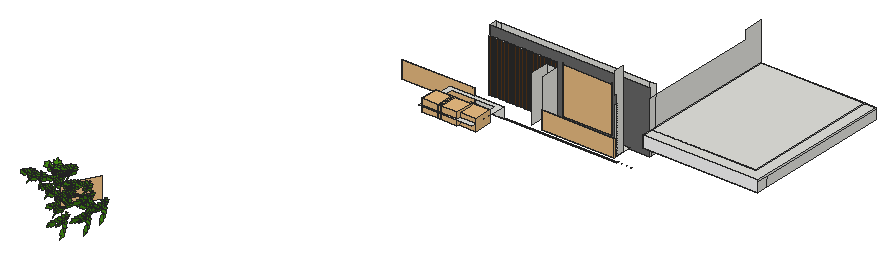
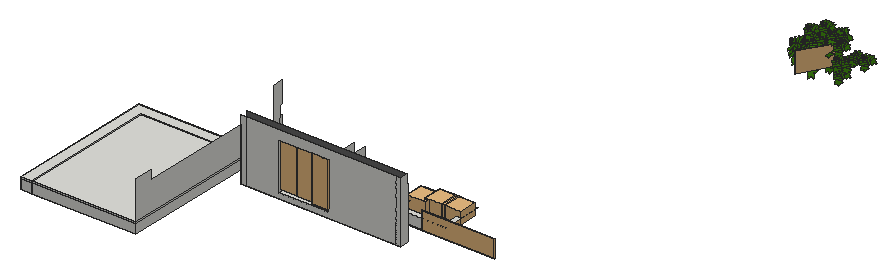
# SketchUp Ruby script. Lengths in inches.
U = 1.inch
M = Sketchup.active_model
def pt(a) = Geom::Point3d.new(a.map { |v| v * U })
def face(e, loops, mat)
  f = e.add_face(loops[0].map { |a| pt(a) })
  loops[1..].each { |l| e.add_face(l.map { |a| pt(a) }).erase! }
  f.material = f.back_material = mat if mat
  f
end
# faces: each face lists its corners as indices into pts; further lists are holes
def faces(e, pts, list, mat = nil) = list.each { |f| face(e, (f[0].is_a?(Array) ? f : [f]).map { |l| l.map { |i| pts[i] } }, mat) }
# xy, xz, yz: faces in a plane at the given z, y or x. An outline is a flat list of corners, or four numbers for a rectangle; further outlines are holes
def ring(l) = l.size == 4 ? [[l[0], l[1]], [l[2], l[1]], [l[2], l[3]], [l[0], l[3]]] : l.each_slice(2).to_a
def flat(e, list, mat, &to3) = list.each { |f| face(e, (f[0].is_a?(Array) ? f : [f]).map { |l| ring(l).map { |u, v| to3.(u, v) } }, mat) }
def xy(e, z, list, mat = nil) = flat(e, list, mat) { |x, y| [x, y, z] }
def xz(e, y, list, mat = nil) = flat(e, list, mat) { |x, z| [x, y, z] }
def yz(e, x, list, mat = nil) = flat(e, list, mat) { |y, z| [x, y, z] }
def lines(e, pts, list) = list.each { |a, b| e.add_line(pt(pts[a]), pt(pts[b])) }
# prism: a flat outline (further loops are holes) pulled along v
def prism(e, loops, v, mat = nil)
  f = face(e, loops, mat); d = Geom::Vector3d.new(v.map { |x| x * U })
  f.pushpull(f.normal.samedirection?(d) ? d.length : -d.length)
end
def box(e, o, s, mat = nil) = prism(e, [[o, [o[0] + s[0], o[1], o[2]], [o[0] + s[0], o[1] + s[1], o[2]], [o[0], o[1] + s[1], o[2]]]], [0, 0, s[2]], mat)
def at(x, y, z, deg = 0) = Geom::Transformation.translation(pt([x, y, z])) * Geom::Transformation.rotation(ORIGIN, Z_AXIS, deg.degrees)
def axes(o, x, y, z) = Geom::Transformation.new([*x, 0, *y, 0, *z, 0, *pt(o).to_a, 1])
def part(name) = M.definitions.add(name)
# library, detail: a bought-in or finely detailed component or shape, given as its bounding box
def library(name, o, s) = part(name).tap { |d| box(d.entities, o, s) }
def detail(e, o, s) = box(e.add_group.entities, o, s)
def put(e, d, t, mat = nil) = e.add_instance(d, t).tap { |i| i.material = mat if mat }
def group(e, t, mat = nil) = e.add_group.tap { |g| g.transformation = t; g.material = mat if mat }.entities
root = M.entities
M.materials.add("Material~3").color = [123, 113, 102]
M.materials.add("[0030_OldLace]").color = [86, 53, 24]
M.materials.add("[0128_White]").color = [255, 255, 255]
M.materials.add("[Slate Light Tile]").color = [104, 104, 104]
M.materials.add("[Wood Veneer 01]").color = [120, 70, 37]
M.materials.add("hojas").color = [70, 150, 19]
c1 = part("rama-acacia")
p = [[-13.53,0.69,-1.07],[-13.38,0.86,-0.98],[-13.61,0.85,-1.06],[-14.07,0.85,-1.21],[-15.17,0.86,-1.58],[-15.95,0.92,-1.83],
  [-16.01,1,-1.83],[-16.01,1.17,-1.78],[-16.07,1.93,-1.6],[-16.4,2.73,-1.5],[-16.65,3.06,-1.5],[-17.13,4.01,-1.41],
  [-17.78,4.7,-1.44],[-18.28,5.07,-1.51],[-18.57,5.18,-1.58],[-18.91,5.47,-1.62],[-19.07,5.48,-1.67],[-19.35,5.61,-1.73],
  [-19.51,5.64,-1.78],[-19.38,5.57,-1.75],[-19.33,5.5,-1.75],[-19.31,5.23,-1.82],[-19.38,5.08,-1.89],[-19.41,4.84,-1.96],
  [-19.36,4.59,-2.01],[-19.43,4.55,-2.04],[-19.36,4.15,-2.125],[-19.21,3.7,-2.19],[-18.875,3.1,-2.24],[-18.61,2.78,-2.24],
  [-17.83,2.19,-2.13],[-17.4375,1.85,-2.09],[-17.04,1.49,-2.05],[-16.61,1.24,-1.97],[-16.17,1.0625,-1.87],[-16.06,0.95,-1.86],
  [-16.06,0.91,-1.87],[-16.32,0.9,-1.96],[-16.7,0.88,-2.1],[-17.05,0.91,-2.21],[-17.61,1.15,-2.33],[-18.06,1.29,-2.45],
  [-18.88,1.53,-2.67],[-20.25,1.46,-3.15],[-20.59,1.49,-3.26],[-20.79,1.37,-3.36],[-21.08,1.2,-3.5],[-21.28,1.22,-3.5625],
  [-21.48,0.94,-3.71],[-21.79,0.5,-3.93],[-22.02,0.17,-4.1],[-22.11,0.05,-4.16],[-22.21,-0.02,-4.21],[-22.375,-0.05,-4.28],
  [-22.375,-0.07,-4.28],[-22.18,-0.09,-4.22],[-22.11,-0.07,-4.19],[-21.78,-0.1,-4.09],[-21.6,-0.18,-4.05],[-21.52,-0.27,-4.04],
  [-21.33,-0.33,-4],[-20.94,-0.54,-3.92],[-20.6875,-0.63,-3.86],[-20.54,-0.68,-3.82],[-20.42,-0.67,-3.78],[-20.09,-0.46,-3.61],
  [-19.8,-0.24,-3.45],[-19.21,-0.02,-3.19],[-18.48,0.08,-2.92],[-17.72,0.38,-2.58],[-17.4,0.5,-2.4375],[-16.93,0.75,-2.21],
  [-16.78,0.8,-2.15],[-16.1,0.83,-1.91],[-16.0625,0.81,-1.9],[-16.08,0.77,-1.91],[-16.27,0.72,-1.99],[-16.88,0.39,-2.29],
  [-17.1875,0.15,-2.46],[-17.27,0.02,-2.52],[-17.94,-0.52,-2.89],[-17.94,-0.59,-2.91],[-18.08,-0.68,-2.99],[-18.13,-0.86,-3.05],
  [-18.56,-1.55,-3.38],[-18.71,-2.11,-3.58],[-18.79,-2.61,-3.74],[-18.86,-2.84,-3.83],[-18.87,-3.07,-3.89],[-18.84,-3.22,-3.92],
  [-18.8,-3.26,-3.92],[-18.76,-3.47,-3.96],[-18.76,-3.6,-4],[-18.67,-3.8,-4.02],[-18.61,-3.92,-4.04],[-18.58,-4.11,-4.07],
  [-18.53,-4.18,-4.08],[-18.58,-4.35,-4.14],[-18.65,-4.43,-4.18],[-18.72,-4.51,-4.23],[-18.8125,-4.51,-4.26],[-18.8125,-4.53,-4.26],
  [-18.72,-4.54,-4.24],[-18.66,-4.49,-4.21],[-18.58,-4.43,-4.16],[-18.35,-4.23,-4.03],[-18.32,-4.17,-4],[-18.22,-4.125,-3.95],
  [-18.1,-4,-3.88],[-17.79,-3.72,-3.7],[-17.68,-3.51,-3.61],[-17.32,-3.13,-3.38],[-17.24,-2.94,-3.31],[-16.78,-2.12,-2.93],
  [-16.48,-1.78,-2.73],[-16.3,-1.28,-2.54],[-16.05,-0.75,-2.3125],[-15.89,-0.2,-2.11],[-15.89,0.39,-1.95],[-15.96,0.79,-1.87],
  [-15.91,0.82,-1.84],[-15.27,0.8,-1.63],[-14.18,0.76,-1.27],[-13.78,0.73,-1.15],[-13.78,0.67,-1.16],[-14.23,0.54,-1.35],
  [-14.65,0.33,-1.55],[-14.97,0.02,-1.74],[-15.25,-0.36,-1.9375],[-15.57,-0.72,-2.14],[-15.96,-1.64,-2.52],[-16.2,-2.51,-2.84],
  [-16.2,-3.12,-3],[-16.14,-3.41,-3.06],[-16.1,-3.75,-3.14],[-16.1,-4.09,-3.23],[-16.2,-4.25,-3.3],[-16.2,-4.28,-3.3125],
  [-16.08,-4.19,-3.24],[-15.98,-4.08,-3.18],[-15.96,-3.94,-3.14],[-15.96,-3.8125,-3.1],[-15.9,-3.72,-3.06],[-15.68,-3.55,-2.9375],
  [-15.51,-3.49,-2.86],[-15.3,-3.33,-2.75],[-15.23,-3.17,-2.68],[-15.01,-3.03,-2.57],[-14.875,-2.83,-2.47],[-14.6,-2.59,-2.3125],
  [-14.4,-2.27,-2.16],[-14.12,-1.6,-1.89],[-13.91,-1.1,-1.68],[-13.67,-0.83,-1.53],[-13.53,-0.45,-1.38],[-13.53,0.67,-1.08],
  [-12.41,6.01,0.65],[-12.44,6.14,0.68],[-12.41,6.29,0.73],[-12.43,6.29,0.73],[-12.44,6.26,0.72],[-12.47,6.15,0.68],
  [-12.49,6.07,0.66],[-12.57,5.75,0.55],[-12.67,5.36,0.43],[-12.79,4.875,0.28],[-12.83,4.52,0.18],[-12.83,3.99,0.04],
  [-12.73,3.11,-0.18],[-12.58,2.52,-0.3125],[-12.3,1.97,-0.41],[-11.88,1.51,-0.46],[-11.37,1.0625,-0.48],[-10.75,0.75,-0.45],
  [-10.75,0.68,-0.47],[-12.55,0.7,-0.79],[-13.21,0.79,-0.89],[-13.2,0.67,-0.92],[-12.56,0.62,-0.82],[-11.15,0.56,-0.58],
  [-10.79,0.54,-0.52],[-10.72,0.52,-0.51],[-10.72,0.5,-0.52],[-10.87,0.47,-0.55],[-11.14,0.41,-0.62],[-11.39,0.27,-0.7],
  [-11.625,-0.01,-0.82],[-11.8,-0.43,-0.96],[-11.83,-0.57,-1],[-12.02,-1.08,-1.17],[-12.1,-1.39,-1.27],[-12.17,-1.95,-1.4375],
  [-12.17,-2.77,-1.65],[-12.09,-3.59,-1.86],[-11.86,-4.26,-2],[-11.8125,-4.4,-2.03],[-11.84,-4.49,-2.05],[-11.91,-4.6,-2.1],
  [-11.97,-4.65,-2.12],[-11.98,-4.67,-2.13],[-11.92,-4.65,-2.11],[-11.84,-4.59,-2.08],[-11.77,-4.52,-2.05],[-11.74,-4.47,-2.03],
  [-11.37,-4.3125,-1.92],[-10.95,-4.0625,-1.78],[-10.82,-3.89,-1.71],[-10.64,-3.57,-1.59],[-10.41,-3.05,-1.41],[-10.27,-2.73,-1.3],
  [-10.07,-1.88,-1.03],[-10.15,-0.71,-0.73],[-10.31,-0.1,-0.6],[-10.5,0.4,-0.5],[-10.5,0.48,-0.48],[-10.44,0.53,-0.45],
  [-10.39,0.64,-0.42],[-10.52,0.73,-0.42],[-10.44,0.93,-0.35],[-10.44,1.2,-0.28],[-10.32,1.47,-0.18],[-10.48,2.6875,0.12],
  [-10.43,2.96,0.2],[-10.75,3.87,0.38],[-11.26,4.93,0.57],[-11.8,5.54,0.64],[-12.37,5.93,0.64],[-7.78,0.19,-0.06],
  [-7.78,0.25,-0.04],[-7.75,0.39,0],[-7.89,0.4,-0.02],[-7.96,0.46,-0.02],[-7.96,0.49,-0.01],[-7.76,0.62,0.06],
  [-7.53,0.99,0.2],[-7.31,1.78,0.45],[-7.31,2.74,0.71],[-7.63,3.6875,0.9],[-8.02,4.57,1.07],[-8.66,5.23,1.13],
  [-8.83,5.4,1.14],[-8.92,5.54,1.16],[-9.1,5.64,1.16],[-9.08,5.6,1.15],[-9.02,5.56,1.15],[-8.94,5.46,1.14],
  [-8.9,5.37,1.12],[-8.9375,5.25,1.08],[-9.14,4.92,0.96],[-9.31,4.5625,0.83],[-9.39,3.73,0.6],[-9.44,2.76,0.32],
  [-9.23,1.59,0.05],[-8.82,0.9,-0.06],[-8.36,0.59,-0.0625],[-8.14,0.51,-0.04],[-8.05,0.48,-0.03],[-8.05,0.46,-0.04],
  [-8.12,0.43,-0.06],[-10.1,0.49,-0.4],[-8.22,0.3125,-0.11],[-8.22,0.25,-0.125],[-8.53,0.13,-0.21],[-8.8,-0.16,-0.34],
  [-8.96,-0.61,-0.49],[-8.96,-0.87,-0.56],[-9.16,-1.42,-0.74],[-9.13,-1.77,-0.83],[-9.09,-1.83,-0.84],[-9.125,-1.92,-0.87],
  [-9.125,-2.13,-0.93],[-9.08,-2.23,-0.95],[-9.15,-2.39,-1],[-9.11,-2.67,-1.07],[-9.03,-2.86,-1.11],[-9.07,-3.03,-1.16],
  [-8.97,-3.23,-1.19],[-8.93,-3.44,-1.24],[-8.93,-3.71,-1.32],[-8.79,-4.05,-1.38],[-8.7,-4.25,-1.42],[-8.7,-4.39,-1.46],
  [-8.76,-4.53,-1.5],[-8.77,-4.65,-1.54],[-8.64,-4.55,-1.49],[-8.27,-4.22,-1.33],[-8.1875,-4.06,-1.27],[-8.07,-3.98,-1.23],
  [-7.98,-3.79,-1.17],[-7.79,-3.59,-1.08],[-7.64,-3.3,-0.97],[-7.64,-3.25,-0.96],[-7.59,-3.21,-0.9375],[-7.52,-2.93,-0.85],
  [-7.52,-2.85,-0.83],[-7.47,-2.81,-0.81],[-7.3,-2.09,-0.59],[-7.32,-2.01,-0.57],[-7.27,-1.95,-0.54],[-7.1875,-1.57,-0.42],
  [-7.17,-1.46,-0.39],[-7.17,-1.16,-0.3125],[-7.23,-0.61,-0.17],[-7.49,-0.15,-0.1],[-13.39,-0.07,-1.23],[-13.39,0.25,-1.14],
  [-13.49,0.5625,-1.09],[-13.8,1.01,-1.08],[-13.61,0.91,-1.04],[-13.38,0.92,-0.96],[-13.32,1.03,-0.91],[-13.32,1.35,-0.82],
  [-13.28,1.49,-0.77],[-13.28,1.99,-0.64],[-13.44,2.67,-0.51],[-13.72,3.31,-0.43],[-13.93,3.71,-0.4],[-14.1,4.39,-0.27],
  [-14.5625,5.06,-0.25],[-14.89,5.62,-0.21],[-15.33,6.1,-0.23],[-15.65,6.8,-0.15],[-15.79,6.89,-0.18],[-15.61,6.52,-0.22],
  [-15.51,6.32,-0.24],[-15.45,6.28,-0.23],[-15.52,6,-0.32],[-15.63,5.6875,-0.45],[-15.77,4.97,-0.68],[-15.7,4.25,-0.85],
  [-15.46,3,-1.11],[-15,2.03,-1.21],[-14.3,1.29,-1.17],[-4.5625,0.33,0.09],[-4.22,0.49,0.13],[-4,0.7,0.1875],
  [-3.86,0.99,0.26],[-3.77,1.41,0.38],[-3.7,1.73,0.46],[-3.77,1.99,0.53],[-3.85,2.17,0.58],[-3.88,2.57,0.6875],
  [-3.98,2.9,0.78],[-4.0625,2.97,0.8],[-4.1,3.14,0.84],[-4.1875,3.25,0.87],[-4.27,3.55,0.95],[-4.31,3.71,0.99],
  [-4.42,3.9,1.04],[-4.625,4.2,1.125],[-4.72,4.39,1.18],[-4.89,4.57,1.23],[-4.98,4.73,1.27],[-5,4.72,1.26],
  [-5.01,4.51,1.21],[-4.96,4.32,1.16],[-4.97,4.27,1.14],[-5.14,3.78,1.01],[-5.3,3.39,0.91],[-5.44,2.76,0.74],
  [-5.5,2.09,0.56],[-5.57,1.78,0.48],[-5.57,1.42,0.38],[-5.57,1.09,0.29],[-5.47,0.72,0.19],[-5.22,0.44,0.12],
  [-4.93,0.27,0.07],[-4.76,0.22,0.06],[-4.76,0.18,0.05],[-4.83,0.16,0.04],[-5.26,0,0],[-5.34,-0.04,-0.01],
  [-5.47,-0.22,-0.06],[-5.51,-0.6,-0.16],[-5.42,-1.09,-0.29],[-5.28,-1.49,-0.4],[-5.21,-1.87,-0.5],[-5.11,-2.15,-0.57],
  [-5.08,-2.34,-0.63],[-5.01,-2.47,-0.66],[-4.96,-2.69,-0.72],[-4.86,-2.9375,-0.79],[-4.84,-3.07,-0.82],[-4.77,-3.18,-0.85],
  [-4.74,-3.43,-0.92],[-4.7,-3.71,-0.99],[-4.62,-3.89,-1.04],[-4.58,-3.98,-1.07],[-4.58,-3.83,-1.03],[-4.51,-3.67,-0.98],
  [-4.3,-3.32,-0.89],[-4.16,-3.09,-0.83],[-4.16,-2.98,-0.8],[-4.11,-2.92,-0.78],[-4.02,-2.8,-0.75],[-3.95,-2.59,-0.69],
  [-3.95,-2.33,-0.625],[-3.86,-2.26,-0.6],[-3.86,-2.02,-0.54],[-3.86,-1.44,-0.39],[-3.94,-1.22,-0.33],[-3.94,-1.08,-0.29],
  [-4,-0.96,-0.26],[-4,-0.87,-0.23],[-4.0625,-0.8125,-0.22],[-4.16,-0.54,-0.14],[-4.39,-0.24,-0.06],[-4.61,-0.08,-0.02],
  [-4.77,-0.03,-0.01],[-4.77,-0.01,0],[-4.65,-0.01,0],[-4.61,0.19,0.05],[-4.66,0.23,0.0625],[-4.63,0.29,0.08],
  [-4.07,0.17,0.04],[0,-0.24,-0.06],[0,0,0],[-0.5,0.04,0.01],[-1.58,0.08,0.02],[-13.78,0.67,-1.08]]
faces(c1.entities,p,[[0,1,2,3,4,5,6,7,8,9,10,11,12,13,14,15,16,17,18,19,20,21,22,23,24,25,26,27,28,29,30,31,32,33,34,35,36,37,38,39,40,41,42,43,44,45,46,47,48,49,50,51,52,53,54,55,56,57,58,59,60,61,62,63,64,65,66,67,68,69,70,71,72,73,74,75,76,77,78,79,80,81,82,83,84,85,86,87,88,89,90,91,92,93,94,95,96,97,98,99,100,101,102,103,104,105,106,107,108,109,110,111,112,113,114,115,116,117,118,119,120,121,122,123,124,125,126,127,128,129,130,131,132,133,134,135,136,137,138,139,140,141,142,143,144,145,146,147,148,149,150,151,152,153,154,155],[156,157,158,159,160,161,162,163,164,165,166,167,168,169,170,171,172,173,174,175,176,177,178,179,180,181,182,183,184,185,186,187,188,189,190,191,192,193,194,195,196,197,198,199,200,201,202,203,204,205,206,207,208,209,210,211,212,213,214,215,216,217,218,219,220,221,222,223,224,225,226],[227,228,229,230,231,232,233,234,235,236,237,238,239,240,241,242,243,244,245,246,247,248,249,250,251,252,253,254,255,256,257,258,216,215,259,260,261,262,263,264,265,266,267,268,269,270,271,272,273,274,275,276,277,278,279,280,281,282,283,284,285,286,287,288,289,290,291,292,293,294,295,296,297,298,299,300,301,302,303],[154,304,305,306,155],[307,308,1,309,310,311,312,313,314,315,316,317,318,319,320,321,322,323,324,325,326,327,328,329,330,331,332],[333,334,335,336,337,338,339,340,341,342,343,344,345,346,347,348,349,350,351,352,353,354,355,356,357,358,359,360,361,362,363,364,365,366,367,368,369,370,371,372,373,374,375,376,377,378,379,380,381,382,383,384,385,386,387,388,389,390,391,392,393,394,395,396,397,398,399,400,401,402,403,404,405,406,407,408,409,410,411,412,413],[0,177,1],[308,2,1],
  [176,1,177],[414,411,410,415,416,417,418],[228,370,229],[369,229,370]],"hojas")
lines(c1.entities,p,[[155,419]])
c2 = part("Group\#150")
put(c2.entities,c1,axes([10.13,10.27,0],[0.45315,0.21131,0],[-0.21131,0.45315,0],[0,0,0.5]))
put(c2.entities,c1,axes([10.13,10.27,0],[0.11638,0.47539,0.10227],[-0.48087,0.12813,-0.0484],[-0.07223,-0.08709,0.48703]))
put(c2.entities,c1,axes([9.58,10.26,-0.7],[0.1449,0.38901,-0.2787],[-0.10883,0.31035,0.37662],[0.46601,-0.04848,0.17461]))
c3 = part("Group\#151")
put(c3.entities,c2,axes([24.99,4.24,9.59],[0.78856,0.61496,0],[0.01473,-0.01889,0.99971],[0.61478,-0.78833,-0.02396]))
put(c3.entities,c2,axes([39.5,6.625,12.55],[0.6544,0.49291,0.57341],[-0.44023,-0.3682,0.81892],[0.61478,-0.78833,-0.02396]))
put(c3.entities,c2,axes([32.34,3.7,6.88],[0.78856,0.61496,0],[0.01473,-0.01889,0.99971],[0.61478,-0.78833,-0.02396]))
put(c3.entities,c2,axes([43.14,6.65,17.54],[0.78856,0.61496,0],[0.35273,-0.4523,0.81915],[0.50374,-0.64595,-0.57358]))
put(c3.entities,c2,axes([12.2,6.2,16.68],[0.7209,0.54936,0.4225],[-0.31991,-0.27701,0.90605],[0.61478,-0.78833,-0.02396]))
put(c3.entities,c2,axes([49.9375,3.79,26.09],[0.78856,0.61496,0],[0.01473,-0.01889,0.99971],[0.61478,-0.78833,-0.02396]))
put(c3.entities,c2,axes([36.11,4.9375,33.94],[0.78856,0.61496,0],[0.01473,-0.01889,0.99971],[0.61478,-0.78833,-0.02396]))
put(c3.entities,c2,axes([39.61,3.79,23.47],[0.78856,0.61496,0],[0.01473,-0.01889,0.99971],[0.61478,-0.78833,-0.02396]))
put(c3.entities,c2,axes([25.59,6.5625,46.47],[-0.40704,-0.29112,-0.86578],[0.67555,0.54201,-0.49986],[0.61478,-0.78833,-0.02396]))
put(c3.entities,c2,axes([54.97,1.98,11.65],[0.78856,0.61496,0],[0.01473,-0.01889,0.99971],[0.61478,-0.78833,-0.02396]))
put(c3.entities,c2,axes([32.97,3.79,19.14],[0.78856,0.61496,0],[0.01473,-0.01889,0.99971],[0.61478,-0.78833,-0.02396]))
put(c3.entities,c2,axes([24.24,3.79,21.99],[0.78856,0.61496,0],[0.01473,-0.01889,0.99971],[0.61478,-0.78833,-0.02396]))
put(c3.entities,c2,axes([16.86,4.24,12.3],[0.78856,0.61496,0],[0.01473,-0.01889,0.99971],[0.61478,-0.78833,-0.02396]))
put(c3.entities,c2,axes([1.23,3.9375,19.07],[0.78856,0.61496,0],[0.01473,-0.01889,0.99971],[0.61478,-0.78833,-0.02396]))
put(c3.entities,c2,axes([29.05,5.25,29.11],[0.78856,0.61496,0],[0.21033,-0.2697,0.93969],[0.57787,-0.741,-0.34202]))
put(c3.entities,c2,axes([24.16,3.79,-0.1],[0.78856,0.61496,0],[0.01473,-0.01889,0.99971],[0.61478,-0.78833,-0.02396]))
c4 = library("Group\#152",[0,0,0],[130.24,0.88,39.6])
c5 = part("glass-railing")
detail(c5.entities,[0,0,0],[1.26,75.59,33.1875])
c6 = library("Ornamental+Grasses",[-8.33,-8.78,0],[17.11,15.88,10.63])
c7 = library("3DGeom~4_Defintion",[362.52,-15.59,12.6],[288.85,70.11,1000])
c8 = library("3 door",[0,0,0],[74.8,3.9375,43.31])
xy(root,162.75,[[3050.93,845.35,3467.75,846.1],[3276.05,888.83,3276.05,890.39,3274.47,890.39,3274.47,888.95,3269.05,888.95,3269.05,890.39,3267.47,890.39,3267.47,888.95,3262.05,888.95,3262.05,890.39,3260.47,890.39,3260.47,888.95,3255.05,888.95,3255.05,890.39,3253.47,890.39,3253.47,888.95,3248.05,888.95,3248.05,890.39,3246.47,890.39,3246.47,888.95,3241.05,888.95,3241.05,890.39,3239.47,890.39,3239.47,888.95,3234.05,888.95,3234.05,890.39,3232.47,890.39,3232.47,888.95,3227.05,888.95,3227.05,890.39,3225.47,890.39,3225.47,888.95,3220.05,888.95,3220.05,890.39,3218.47,890.39,3218.47,888.95,3213.05,888.95,3213.05,890.39,3211.47,890.39,3211.47,888.95,3206.05,888.95,3206.05,890.39,3204.47,890.39,3204.47,888.95,3199.05,888.95,3199.05,890.39,3197.47,890.39,3197.47,888.95,3192.05,888.95,3192.05,890.39,3190.41,890.39,3190.41,888.95,3184.99,888.95,3184.99,905.7,3496.96,905.7,3496.96,890.39,3316.47,890.39,3316.47,888.83,3311.05,888.83,3311.05,890.39,3309.47,890.39,3309.47,888.83,3304.05,888.83,3304.05,890.39,3302.47,890.39,3302.47,888.83,3297.05,888.83,3297.05,890.39,3295.47,890.39,3295.47,888.83,3290.05,888.83,3290.05,890.39,3288.47,890.39,3288.47,888.83,3283.05,888.83,3283.05,890.39,3281.47,890.39,3281.47,888.83]])
xy(root,163,[[3467.75,845.35,3496.96,846.1]])
xy(root,173.4375,[[3327.33,840.97,3467.75,877.14],[3327.52,890.39,3422.58,905.7]])
xy(root,183.3125,[[[3145.18,767.72,3249.37,845.35],[3153.83,776.37,3240.72,836.7]]])
xy(root,186.75,[[3683.87,893.65,3690.02,895.71],[3692.18,893.65,3698.33,895.71],[3501,894.34,3507.14,895.71],[3509.31,894.34,3515.46,895.71],[3517.62,894.34,3523.77,895.71],
  [3525.93,894.34,3532.08,895.71],[3534.25,894.34,3540.39,895.71],[3542.56,894.34,3548.71,895.71],[3550.87,894.34,3557.02,895.71],[3559.18,894.34,3565.33,895.71],
  [3567.5,894.34,3573.64,895.71],[3575.81,894.34,3581.96,895.71],[3584.12,894.34,3590.27,895.71],[3592.43,894.34,3598.58,895.71],[3600.75,894.34,3606.89,895.71],
  [3609.06,894.34,3615.21,895.71],[3617.37,894.34,3623.52,895.71],[3625.68,894.34,3631.83,895.71],[3634,894.34,3640.14,895.71],[3642.31,894.34,3648.46,895.71],
  [3650.62,894.34,3656.77,895.71],[3658.93,894.34,3665.08,895.71],[3667.25,894.34,3673.39,895.71],[3675.56,894.34,3681.71,895.71],[[3496.96,895.71,3698.33,1160.85],[3505.43,904.18,3687.11,1152.375]]])
xy(root,186.75,[[3496.96,873.28,3496.96,895.71,3501,895.71,3501,894.34,3507.14,894.34,3507.14,895.71,3509.31,895.71,3509.31,894.34,3515.46,894.34,3515.46,895.71,3517.62,895.71,3517.62,894.34,3523.77,894.34,3523.77,895.71,3525.93,895.71,3525.93,894.34,3532.08,894.34,3532.08,895.71,3534.25,895.71,3534.25,894.34,3540.39,894.34,3540.39,895.71,3542.56,895.71,3542.56,894.34,3548.71,894.34,3548.71,895.71,3550.87,895.71,3550.87,894.34,3557.02,894.34,3557.02,895.71,3559.18,895.71,3559.18,894.34,3565.33,894.34,3565.33,895.71,3567.5,895.71,3567.5,894.34,3573.64,894.34,3573.64,895.71,3575.81,895.71,3575.81,894.34,3581.96,894.34,3581.96,895.71,3584.12,895.71,3584.12,894.34,3590.27,894.34,3590.27,895.71,3592.43,895.71,3592.43,894.34,3598.58,894.34,3598.58,895.71,3600.75,895.71,3600.75,894.34,3606.89,894.34,3606.89,895.71,3609.06,895.71,3609.06,894.34,3615.21,894.34,3615.21,895.71,3617.37,895.71,3617.37,894.34,3623.52,894.34,3623.52,895.71,3625.68,895.71,3625.68,894.34,3631.83,894.34,3631.83,895.71,3634,895.71,3634,894.34,3640.14,894.34,3640.14,895.71,3642.31,895.71,3642.31,894.34,3648.46,894.34,3648.46,895.71,3650.62,895.71,3650.62,894.34,3656.77,894.34,3656.77,895.71,3658.93,895.71,3658.93,894.34,3665.08,894.34,3665.08,895.71,3667.25,895.71,3667.25,894.34,3673.39,894.34,3673.39,895.71,3675.56,895.71,3675.56,894.34,3681.71,894.34,3681.71,895.71,3683.87,895.71,3683.87,893.65,3690.02,893.65,3690.02,895.71,3692.18,895.71,3692.18,893.65,3698.33,893.65,3698.33,895.71,3720.76,895.71,3720.76,873.28],[3698.33,895.71,3720.76,1160.85]],"[Wood Veneer 01]")
xy(root,204.8125,[[[3496.96,895.71,3698.33,1160.85],[3505.43,904.18,3687.11,1152.375]],[3698.33,895.71,3720.76,1160.85]])
xy(root,208.375,[[3496.96,873.28,3720.76,873.28,3720.76,1160.85,3698.33,1160.85,3698.33,895.71,3496.96,895.71],[3496.96,895.71,3698.33,1160.85]])
xz(root,845.35,[[3145.18,162.75,3249.37,183.3125]])
xz(root,873.28,[[3496.96,186.75,3720.76,208.375]],"[0128_White]")
xz(root,877.14,[[3307.68,173.4375,3327.33,264.75]])
xz(root,888.83,[[3276.05,162.75,3281.47,264.75],[3283.05,162.75,3288.47,264.75],[3290.05,162.75,3295.47,264.75],[3297.05,162.75,3302.47,264.75],[3304.05,162.75,3309.47,264.75],
  [3311.05,162.75,3316.47,264.75]],"[0030_OldLace]")
xz(root,888.95,[[3184.99,162.75,3190.41,264.75],[3192.05,162.75,3197.47,264.75],[3199.05,162.75,3204.47,264.75],[3206.05,162.75,3211.47,264.75],[3213.05,162.75,3218.47,264.75],
  [3220.05,162.75,3225.47,264.75],[3227.05,162.75,3232.47,264.75],[3234.05,162.75,3239.47,264.75],[3241.05,162.75,3246.47,264.75],[3248.05,162.75,3253.47,264.75],
  [3255.05,162.75,3260.47,264.75],[3262.05,162.75,3267.47,264.75],[3269.05,162.75,3274.47,264.75]],"[0030_OldLace]")
xz(root,890.39,[[[3190.41,162.75,3192.05,162.75,3192.05,264.75,3197.47,264.75,3197.47,162.75,3199.05,162.75,3199.05,264.75,3204.47,264.75,3204.47,162.75,3206.05,162.75,3206.05,264.75,3211.47,264.75,3211.47,162.75,3213.05,162.75,3213.05,264.75,3218.47,264.75,3218.47,162.75,3220.05,162.75,3220.05,264.75,3225.47,264.75,3225.47,162.75,3227.05,162.75,3227.05,264.75,3232.47,264.75,3232.47,162.75,3234.05,162.75,3234.05,264.75,3239.47,264.75,3239.47,162.75,3241.05,162.75,3241.05,264.75,3246.47,264.75,3246.47,162.75,3248.05,162.75,3248.05,264.75,3253.47,264.75,3253.47,162.75,3255.05,162.75,3255.05,264.75,3260.47,264.75,3260.47,162.75,3262.05,162.75,3262.05,264.75,3267.47,264.75,3267.47,162.75,3269.05,162.75,3269.05,264.75,3274.47,264.75,3274.47,162.75,3276.05,162.75,3276.05,264.75,3281.47,264.75,3281.47,162.75,3283.05,162.75,3283.05,264.75,3288.47,264.75,3288.47,162.75,3290.05,162.75,3290.05,264.75,3295.47,264.75,3295.47,162.75,3297.05,162.75,3297.05,264.75,3302.47,264.75,3302.47,162.75,3304.05,162.75,3304.05,264.75,3309.47,264.75,3309.47,162.75,3311.05,162.75,3311.05,264.75,3316.47,264.75,3316.47,162.75,3496.96,162.75,3496.96,282.75,3184.99,282.75,3184.99,264.75,3190.41,264.75],[3327.52,173.4375,3422.58,264.75]]],"[Slate Light Tile]")
xz(root,895.71,[[3496.96,186.75,3698.33,204.8125],[3698.33,186.75,3720.76,204.8125],[3496.96,204.8125,3698.33,208.375]])
xz(root,904.18,[[3505.43,186.75,3687.11,204.8125]])
xz(root,905.7,[[3184.99,162.75,3194.375,282.75],[[3194.375,162.75,3484.69,282.75],[3327.52,173.4375,3422.58,264.75]],[3484.69,162.75,3496.96,282.75]])
xz(root,1152.375,[[3505.43,186.75,3687.11,204.8125]])
xz(root,1160.85,[[3496.96,186.75,3698.33,204.8125],[3698.33,186.75,3720.76,204.8125],[3496.96,204.8125,3698.33,208.375],[3698.33,204.8125,3720.76,208.375]])
yz(root,3184.99,[[888.95,162.75,888.95,264.75,890.39,264.75,890.39,282.75,905.7,282.75,905.7,162.75]])
yz(root,3190.41,[[888.95,162.75,890.39,264.75]])
yz(root,3192.05,[[888.95,162.75,890.39,264.75]])
yz(root,3197.47,[[888.95,162.75,890.39,264.75]])
yz(root,3199.05,[[888.95,162.75,890.39,264.75]])
yz(root,3204.47,[[888.95,162.75,890.39,264.75]])
yz(root,3206.05,[[888.95,162.75,890.39,264.75]])
yz(root,3211.47,[[888.95,162.75,890.39,264.75]])
yz(root,3213.05,[[888.95,162.75,890.39,264.75]])
yz(root,3218.47,[[888.95,162.75,890.39,264.75]])
yz(root,3220.05,[[888.95,162.75,890.39,264.75]])
yz(root,3225.47,[[888.95,162.75,890.39,264.75]])
yz(root,3227.05,[[888.95,162.75,890.39,264.75]])
yz(root,3232.47,[[888.95,162.75,890.39,264.75]])
yz(root,3234.05,[[888.95,162.75,890.39,264.75]])
yz(root,3239.47,[[888.95,162.75,890.39,264.75]])
yz(root,3241.05,[[888.95,162.75,890.39,264.75]])
yz(root,3246.47,[[888.95,162.75,890.39,264.75]])
yz(root,3248.05,[[888.95,162.75,890.39,264.75]])
yz(root,3253.47,[[888.95,162.75,890.39,264.75]])
yz(root,3255.05,[[888.95,162.75,890.39,264.75]])
yz(root,3260.47,[[888.95,162.75,890.39,264.75]])
yz(root,3262.05,[[888.95,162.75,890.39,264.75]])
yz(root,3267.47,[[888.95,162.75,890.39,264.75]])
yz(root,3269.05,[[888.95,162.75,890.39,264.75]])
yz(root,3274.47,[[888.95,162.75,890.39,264.75]])
yz(root,3276.05,[[888.83,162.75,890.39,264.75]])
yz(root,3281.47,[[888.83,162.75,890.39,264.75]])
yz(root,3283.05,[[888.83,162.75,890.39,264.75]])
yz(root,3288.47,[[888.83,162.75,890.39,264.75]])
yz(root,3290.05,[[888.83,162.75,890.39,264.75]],"[0030_OldLace]")
yz(root,3295.47,[[888.83,162.75,890.39,264.75]])
yz(root,3297.05,[[888.83,162.75,890.39,264.75]],"[0030_OldLace]")
yz(root,3302.47,[[888.83,162.75,890.39,264.75]])
yz(root,3304.05,[[888.83,162.75,890.39,264.75]],"[0030_OldLace]")
yz(root,3307.68,[[840.97,173.4375,877.14,264.75]])
yz(root,3309.47,[[888.83,162.75,890.39,264.75]])
yz(root,3311.05,[[888.83,162.75,890.39,264.75]],"[0030_OldLace]")
yz(root,3316.47,[[888.83,162.75,890.39,264.75]])
yz(root,3327.33,[[840.97,173.4375,877.14,264.75]])
yz(root,3327.52,[[890.39,173.4375,905.7,264.75]])
yz(root,3422.58,[[890.39,173.4375,905.7,264.75]])
yz(root,3467.75,[[845.35,162.75,846.1,163],[840.97,173.4375,846.1,264.75],[846.1,173.4375,846.1,264.75,845.35,264.75,845.35,282.75,840.97,282.75,840.97,324.5625,861.24,324.5625,861.24,173.4375]])
yz(root,3496.96,[[890.39,162.75,895.71,186.75],[895.71,162.75,905.7,186.75],[873.28,186.75,890.39,204.8125],[890.39,186.75,895.71,204.8125],[895.71,186.75,905.7,204.8125],
  [905.7,186.75,1160.85,204.8125],[873.28,204.8125,890.39,208.375],[890.39,204.8125,895.71,208.375],[895.71,204.8125,905.7,208.375],[905.7,204.8125,1160.85,208.375],
  [890.39,208.375,905.7,264.75],[905.7,208.375,1160.85,208.375,1160.85,282.75,1122.97,282.75,1122.97,264.75,905.7,264.75]])
yz(root,3505.43,[[904.18,186.75,905.7,204.8125],[905.7,186.75,1152.375,204.8125]])
yz(root,3687.11,[[904.18,186.75,1152.375,204.8125]])
yz(root,3698.33,[[895.71,186.75,1160.85,204.8125],[895.71,204.8125,1160.85,208.375]])
yz(root,3720.76,[[873.28,186.75,895.71,204.8125],[895.71,186.75,1160.85,204.8125],[873.28,204.8125,1160.85,208.375]])
p = [[3319.625,890.39,264.75],[3319.625,890.39,162.75]]
lines(root,p,[[0,1]])
put(root,c3,axes([2878.69,120.89,195.34],[2.21,0,0],[0,2.21,0],[0,0,2.21]))
put(root,c4,axes([2989.92,190.85,218.68],[-0.25572,-0.42966,0],[0.17186,-0.10229,0],[0,0,1]))
put(root,c2,axes([2995.33,54.97,209.18],[0.37045,4.09667,0],[0.08998,-0.06733,3.00354],[3.7549,-2.80958,-0.07198]))
put(root,c2,axes([2998.73,108.11,194.02],[0.37045,4.09667,0],[0.08998,-0.06733,3.00354],[3.7549,-2.80958,-0.07198]))
put(root,c2,axes([2999.68,111.5,223.15],[0.37045,4.09667,0],[0.08998,-0.06733,3.00354],[3.7549,-2.80958,-0.07198]))
put(root,c2,axes([3020.26,119.96,215.01],[0.37045,4.09667,0],[0.08998,-0.06733,3.00354],[3.7549,-2.80958,-0.07198]))
put(root,c5,axes([3051.87,845.7,162.75],[0,-1,0],[1.87,0,0],[0,0,1]))
put(root,c6,axes([3165.34,791.57,170.63],[2.19,0,0],[0,2.19,0],[0,0,2.19]))
put(root,c6,axes([3197.15,791.57,170.63],[2.19,0,0],[0,2.19,0],[0,0,2.19]))
put(root,c6,axes([3228.3,798.1875,167.75],[2.19,0,0],[0,2.19,0],[0,0,2.19]))
put(root,c7,axes([3285.66,905.3125,176.31],[0.11056,0,0],[0,-0.05859,0],[0,0,0.08734]),"Material~3")
put(root,c7,axes([3317.26,901.24,176.31],[0.11056,0,0],[0,-0.05859,0],[0,0,0.08734]),"Material~3")
put(root,c8,axes([3327.52,890.39,173.4375],[1.27084,0,0],[0,1.38,0],[0,0,2.15904]))
put(root,c5,axes([3327.27,841,173.4375],[0,-1,0],[1.86,0,0],[0,0,1]))
put(root,c7,axes([3350.57,901.24,176.31],[0.11056,0,0],[0,-0.05859,0],[0,0,0.08734]),"Material~3")
